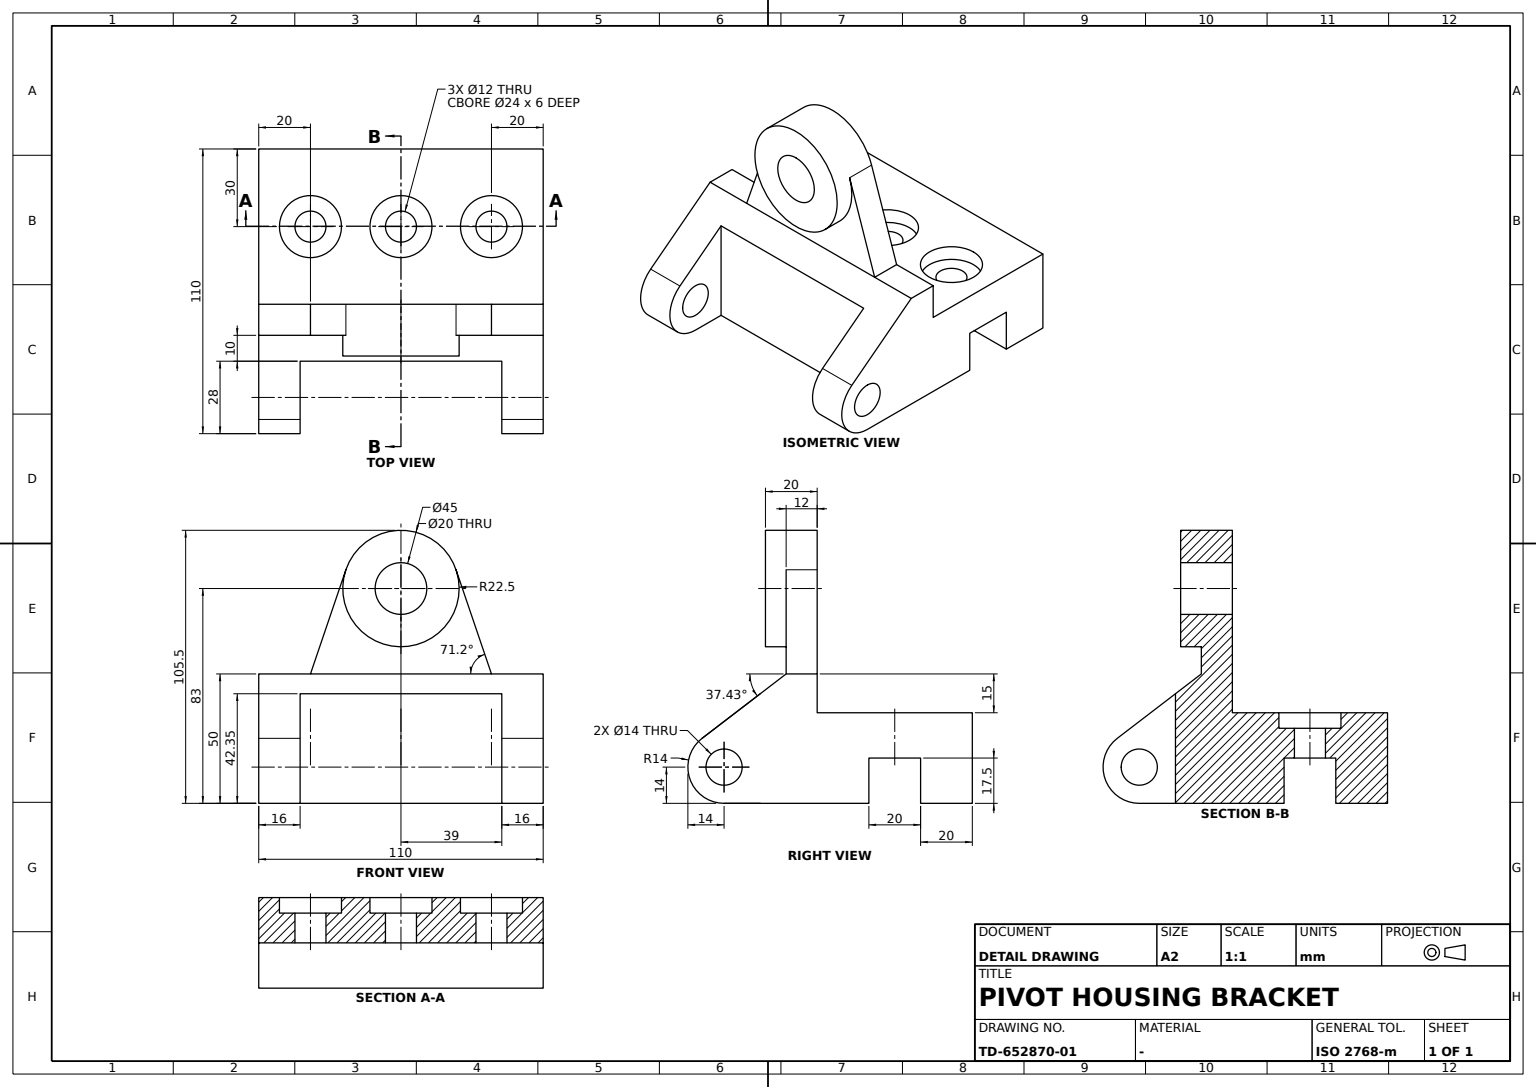
ISO-10303-21;
HEADER;
FILE_DESCRIPTION((''),'2;1');
FILE_NAME('','',(''),(''),'','','');
FILE_SCHEMA(('AUTOMOTIVE_DESIGN'));
ENDSEC;
DATA;
#1=APPLICATION_CONTEXT('');
#2=PRODUCT_CONTEXT('',#1,'mechanical');
#3=PRODUCT('','','',(#2));
#4=PRODUCT_DEFINITION_FORMATION('','',#3);
#5=PRODUCT_DEFINITION_CONTEXT('',#1,'design');
#6=PRODUCT_DEFINITION('','',#4,#5);
#7=PRODUCT_DEFINITION_SHAPE('','',#6);
#8=(LENGTH_UNIT()NAMED_UNIT(*)SI_UNIT(.MILLI.,.METRE.));
#9=(NAMED_UNIT(*)PLANE_ANGLE_UNIT()SI_UNIT($,.RADIAN.));
#10=(NAMED_UNIT(*)SI_UNIT($,.STERADIAN.)SOLID_ANGLE_UNIT());
#11=UNCERTAINTY_MEASURE_WITH_UNIT(LENGTH_MEASURE(0.005),#8,'distance_accuracy_value','');
#12=(GEOMETRIC_REPRESENTATION_CONTEXT(3)GLOBAL_UNCERTAINTY_ASSIGNED_CONTEXT((#11))GLOBAL_UNIT_ASSIGNED_CONTEXT((#8,#9,#10))REPRESENTATION_CONTEXT('',''));
#13=CARTESIAN_POINT('',(35.,-32.,32.5));
#14=VERTEX_POINT('',#13);
#15=CARTESIAN_POINT('',(-35.,-32.,32.5));
#16=VERTEX_POINT('',#15);
#17=DIRECTION('',(-1.,0.,0.));
#18=VECTOR('',#17,1000.);
#19=LINE('',#13,#18);
#20=EDGE_CURVE('',#14,#16,#19,.T.);
#21=ORIENTED_EDGE('',*,*,#20,.F.);
#22=CARTESIAN_POINT('',(21.299957,-32.,72.749954));
#23=VERTEX_POINT('',#22);
#24=DIRECTION('',(0.32222019,0.,-0.94666475));
#25=VECTOR('',#24,1000.);
#26=LINE('',#22,#25);
#27=EDGE_CURVE('',#23,#14,#26,.T.);
#28=ORIENTED_EDGE('',*,*,#27,.F.);
#29=CARTESIAN_POINT('',(-21.299957,-32.,72.749954));
#30=VERTEX_POINT('',#29);
#31=CARTESIAN_POINT('',(0.,-32.,65.5));
#32=DIRECTION('',(0.,1.,0.));
#33=DIRECTION('',(0.,0.,1.));
#34=AXIS2_PLACEMENT_3D('',#31,#32,#33);
#35=CIRCLE('',#34,22.5);
#36=EDGE_CURVE('',#30,#23,#35,.F.);
#37=ORIENTED_EDGE('',*,*,#36,.F.);
#38=DIRECTION('',(0.32222019,0.,0.94666475));
#39=VECTOR('',#38,1000.);
#40=LINE('',#15,#39);
#41=EDGE_CURVE('',#16,#30,#40,.T.);
#42=ORIENTED_EDGE('',*,*,#41,.F.);
#43=EDGE_LOOP('',(#21,#28,#37,#42));
#44=FACE_BOUND('',#43,.T.);
#45=PLANE('',#34);
#46=ADVANCED_FACE('',(#44),#45,.F.);
#47=CARTESIAN_POINT('',(55.,40.,17.5));
#48=VERTEX_POINT('',#47);
#49=CARTESIAN_POINT('',(-55.,40.,17.5));
#50=VERTEX_POINT('',#49);
#51=LINE('',#47,#18);
#52=EDGE_CURVE('',#48,#50,#51,.T.);
#53=ORIENTED_EDGE('',*,*,#52,.F.);
#54=CARTESIAN_POINT('',(55.,40.,-17.5));
#55=VERTEX_POINT('',#54);
#56=DIRECTION('',(0.,0.,-1.));
#57=VECTOR('',#56,1000.);
#58=LINE('',#47,#57);
#59=EDGE_CURVE('',#48,#55,#58,.T.);
#60=ORIENTED_EDGE('',*,*,#59,.T.);
#61=CARTESIAN_POINT('',(-55.,40.,-17.5));
#62=VERTEX_POINT('',#61);
#63=LINE('',#54,#18);
#64=EDGE_CURVE('',#55,#62,#63,.T.);
#65=ORIENTED_EDGE('',*,*,#64,.T.);
#66=LINE('',#49,#57);
#67=EDGE_CURVE('',#50,#62,#66,.T.);
#68=ORIENTED_EDGE('',*,*,#67,.F.);
#69=EDGE_LOOP('',(#53,#60,#65,#68));
#70=FACE_BOUND('',#69,.T.);
#71=AXIS2_PLACEMENT_3D('',#47,#32,#33);
#72=PLANE('',#71);
#73=ADVANCED_FACE('',(#70),#72,.T.);
#74=CARTESIAN_POINT('',(22.5,-40.,65.5));
#75=VERTEX_POINT('',#74);
#76=CARTESIAN_POINT('',(0.,-40.,65.5));
#77=DIRECTION('',(0.,-1.,0.));
#78=DIRECTION('',(1.,0.,0.));
#79=AXIS2_PLACEMENT_3D('',#76,#77,#78);
#80=CIRCLE('',#79,22.5);
#81=EDGE_CURVE('',#75,#75,#80,.T.);
#82=ORIENTED_EDGE('',*,*,#81,.T.);
#83=EDGE_LOOP('',(#82));
#84=FACE_BOUND('',#83,.T.);
#85=CARTESIAN_POINT('',(0.,-40.,75.5));
#86=VERTEX_POINT('',#85);
#87=AXIS2_PLACEMENT_3D('',#76,#32,#33);
#88=CIRCLE('',#87,10.);
#89=EDGE_CURVE('',#86,#86,#88,.T.);
#90=ORIENTED_EDGE('',*,*,#89,.T.);
#91=EDGE_LOOP('',(#90));
#92=FACE_BOUND('',#91,.T.);
#93=AXIS2_PLACEMENT_3D('',#76,#77,#56);
#94=PLANE('',#93);
#95=ADVANCED_FACE('',(#84,#92),#94,.T.);
#96=CARTESIAN_POINT('',(0.,-20.,75.5));
#97=VERTEX_POINT('',#96);
#98=CARTESIAN_POINT('',(0.,-20.,65.5));
#99=AXIS2_PLACEMENT_3D('',#98,#32,#33);
#100=CIRCLE('',#99,10.);
#101=EDGE_CURVE('',#97,#97,#100,.T.);
#102=ORIENTED_EDGE('',*,*,#101,.T.);
#103=EDGE_LOOP('',(#102));
#104=FACE_BOUND('',#103,.T.);
#105=ORIENTED_EDGE('',*,*,#89,.F.);
#106=EDGE_LOOP('',(#105));
#107=FACE_BOUND('',#106,.T.);
#108=CYLINDRICAL_SURFACE('',#87,10.);
#109=ADVANCED_FACE('',(#104,#107),#108,.F.);
#110=CARTESIAN_POINT('',(-21.299957,-20.,72.749954));
#111=VERTEX_POINT('',#110);
#112=VECTOR('',#32,1000.);
#113=LINE('',#29,#112);
#114=EDGE_CURVE('',#30,#111,#113,.T.);
#115=ORIENTED_EDGE('',*,*,#114,.F.);
#116=ORIENTED_EDGE('',*,*,#36,.T.);
#117=CARTESIAN_POINT('',(21.299957,-20.,72.749954));
#118=VERTEX_POINT('',#117);
#119=LINE('',#22,#112);
#120=EDGE_CURVE('',#23,#118,#119,.T.);
#121=ORIENTED_EDGE('',*,*,#120,.T.);
#122=AXIS2_PLACEMENT_3D('',#98,#32,#78);
#123=CIRCLE('',#122,22.5);
#124=EDGE_CURVE('',#111,#118,#123,.T.);
#125=ORIENTED_EDGE('',*,*,#124,.F.);
#126=EDGE_LOOP('',(#115,#116,#121,#125));
#127=FACE_BOUND('',#126,.T.);
#128=ORIENTED_EDGE('',*,*,#81,.F.);
#129=EDGE_LOOP('',(#128));
#130=FACE_BOUND('',#129,.T.);
#131=CYLINDRICAL_SURFACE('',#34,22.5);
#132=ADVANCED_FACE('',(#127,#130),#131,.T.);
#133=CARTESIAN_POINT('',(-39.,-42.,24.84594));
#134=VERTEX_POINT('',#133);
#135=CARTESIAN_POINT('',(-39.,-64.509212,7.617253));
#136=VERTEX_POINT('',#135);
#137=DIRECTION('',(0.,-0.794089474,-0.607800878));
#138=VECTOR('',#137,1000.);
#139=LINE('',#135,#138);
#140=EDGE_CURVE('',#134,#136,#139,.T.);
#141=ORIENTED_EDGE('',*,*,#140,.T.);
#142=CARTESIAN_POINT('',(-39.,-56.,-17.5));
#143=VERTEX_POINT('',#142);
#144=CARTESIAN_POINT('',(-39.,-56.,-3.5));
#145=AXIS2_PLACEMENT_3D('',#144,#17,#77);
#146=CIRCLE('',#145,14.);
#147=EDGE_CURVE('',#136,#143,#146,.F.);
#148=ORIENTED_EDGE('',*,*,#147,.T.);
#149=CARTESIAN_POINT('',(-39.,-42.,-17.5));
#150=VERTEX_POINT('',#149);
#151=CARTESIAN_POINT('',(-39.,-20.,-17.5));
#152=LINE('',#151,#112);
#153=EDGE_CURVE('',#143,#150,#152,.T.);
#154=ORIENTED_EDGE('',*,*,#153,.T.);
#155=CARTESIAN_POINT('',(-39.,-42.,55.));
#156=LINE('',#155,#57);
#157=EDGE_CURVE('',#150,#134,#156,.F.);
#158=ORIENTED_EDGE('',*,*,#157,.T.);
#159=EDGE_LOOP('',(#141,#148,#154,#158));
#160=FACE_BOUND('',#159,.T.);
#161=CARTESIAN_POINT('',(-39.,-63.,-3.5));
#162=VERTEX_POINT('',#161);
#163=CIRCLE('',#145,7.);
#164=EDGE_CURVE('',#162,#162,#163,.T.);
#165=ORIENTED_EDGE('',*,*,#164,.T.);
#166=EDGE_LOOP('',(#165));
#167=FACE_BOUND('',#166,.T.);
#168=CARTESIAN_POINT('',(-39.,-72.,55.));
#169=AXIS2_PLACEMENT_3D('',#168,#17,#77);
#170=PLANE('',#169);
#171=ADVANCED_FACE('',(#160,#167),#170,.F.);
#172=CARTESIAN_POINT('',(6.,10.,0.));
#173=VERTEX_POINT('',#172);
#174=CARTESIAN_POINT('',(0.,10.,0.));
#175=AXIS2_PLACEMENT_3D('',#174,#33,#78);
#176=CIRCLE('',#175,6.);
#177=EDGE_CURVE('',#173,#173,#176,.T.);
#178=ORIENTED_EDGE('',*,*,#177,.F.);
#179=EDGE_LOOP('',(#178));
#180=FACE_BOUND('',#179,.T.);
#181=CARTESIAN_POINT('',(0.,16.,11.5));
#182=VERTEX_POINT('',#181);
#183=CARTESIAN_POINT('',(0.,10.,11.5));
#184=AXIS2_PLACEMENT_3D('',#183,#56,#32);
#185=CIRCLE('',#184,6.);
#186=EDGE_CURVE('',#182,#182,#185,.F.);
#187=ORIENTED_EDGE('',*,*,#186,.T.);
#188=EDGE_LOOP('',(#187));
#189=FACE_BOUND('',#188,.T.);
#190=CARTESIAN_POINT('',(0.,10.,-65.061518));
#191=AXIS2_PLACEMENT_3D('',#190,#56,#32);
#192=CYLINDRICAL_SURFACE('',#191,6.);
#193=ADVANCED_FACE('',(#180,#189),#192,.F.);
#194=CARTESIAN_POINT('',(35.,-20.,32.5));
#195=VERTEX_POINT('',#194);
#196=LINE('',#13,#112);
#197=EDGE_CURVE('',#14,#195,#196,.T.);
#198=ORIENTED_EDGE('',*,*,#197,.T.);
#199=LINE('',#117,#25);
#200=EDGE_CURVE('',#118,#195,#199,.T.);
#201=ORIENTED_EDGE('',*,*,#200,.F.);
#202=ORIENTED_EDGE('',*,*,#120,.F.);
#203=ORIENTED_EDGE('',*,*,#27,.T.);
#204=EDGE_LOOP('',(#198,#201,#202,#203));
#205=FACE_BOUND('',#204,.T.);
#206=DIRECTION('',(0.94666475,0.,0.32222019));
#207=AXIS2_PLACEMENT_3D('',#22,#206,#24);
#208=PLANE('',#207);
#209=ADVANCED_FACE('',(#205),#208,.T.);
#210=CARTESIAN_POINT('',(55.,20.,0.));
#211=VERTEX_POINT('',#210);
#212=CARTESIAN_POINT('',(-55.,20.,0.));
#213=VERTEX_POINT('',#212);
#214=CARTESIAN_POINT('',(75.,20.,0.));
#215=LINE('',#214,#18);
#216=EDGE_CURVE('',#211,#213,#215,.T.);
#217=ORIENTED_EDGE('',*,*,#216,.T.);
#218=CARTESIAN_POINT('',(-55.,20.,-17.5));
#219=VERTEX_POINT('',#218);
#220=LINE('',#212,#57);
#221=EDGE_CURVE('',#219,#213,#220,.F.);
#222=ORIENTED_EDGE('',*,*,#221,.F.);
#223=CARTESIAN_POINT('',(55.,20.,-17.5));
#224=VERTEX_POINT('',#223);
#225=CARTESIAN_POINT('',(75.,20.,-17.5));
#226=LINE('',#225,#18);
#227=EDGE_CURVE('',#224,#219,#226,.T.);
#228=ORIENTED_EDGE('',*,*,#227,.F.);
#229=LINE('',#210,#57);
#230=EDGE_CURVE('',#224,#211,#229,.F.);
#231=ORIENTED_EDGE('',*,*,#230,.T.);
#232=EDGE_LOOP('',(#217,#222,#228,#231));
#233=FACE_BOUND('',#232,.T.);
#234=AXIS2_PLACEMENT_3D('',#225,#32,#33);
#235=PLANE('',#234);
#236=ADVANCED_FACE('',(#233),#235,.F.);
#237=CARTESIAN_POINT('',(-29.,10.,0.));
#238=VERTEX_POINT('',#237);
#239=CARTESIAN_POINT('',(-35.,10.,0.));
#240=AXIS2_PLACEMENT_3D('',#239,#33,#78);
#241=CIRCLE('',#240,6.);
#242=EDGE_CURVE('',#238,#238,#241,.T.);
#243=ORIENTED_EDGE('',*,*,#242,.F.);
#244=EDGE_LOOP('',(#243));
#245=FACE_BOUND('',#244,.T.);
#246=CARTESIAN_POINT('',(-41.,10.,11.5));
#247=VERTEX_POINT('',#246);
#248=CARTESIAN_POINT('',(-35.,10.,11.5));
#249=AXIS2_PLACEMENT_3D('',#248,#56,#17);
#250=CIRCLE('',#249,6.);
#251=EDGE_CURVE('',#247,#247,#250,.F.);
#252=ORIENTED_EDGE('',*,*,#251,.T.);
#253=EDGE_LOOP('',(#252));
#254=FACE_BOUND('',#253,.T.);
#255=CARTESIAN_POINT('',(-35.,10.,-58.75745));
#256=AXIS2_PLACEMENT_3D('',#255,#56,#17);
#257=CYLINDRICAL_SURFACE('',#256,6.);
#258=ADVANCED_FACE('',(#245,#254),#257,.F.);
#259=CARTESIAN_POINT('',(-35.,-20.,32.5));
#260=VERTEX_POINT('',#259);
#261=CARTESIAN_POINT('',(-55.,-20.,32.5));
#262=VERTEX_POINT('',#261);
#263=CARTESIAN_POINT('',(55.,-20.,32.5));
#264=LINE('',#263,#18);
#265=EDGE_CURVE('',#260,#262,#264,.T.);
#266=ORIENTED_EDGE('',*,*,#265,.T.);
#267=CARTESIAN_POINT('',(-55.,-32.,32.5));
#268=VERTEX_POINT('',#267);
#269=LINE('',#267,#112);
#270=EDGE_CURVE('',#268,#262,#269,.T.);
#271=ORIENTED_EDGE('',*,*,#270,.F.);
#272=CARTESIAN_POINT('',(55.,-32.,32.5));
#273=LINE('',#272,#18);
#274=EDGE_CURVE('',#16,#268,#273,.T.);
#275=ORIENTED_EDGE('',*,*,#274,.F.);
#276=LINE('',#15,#112);
#277=EDGE_CURVE('',#16,#260,#276,.T.);
#278=ORIENTED_EDGE('',*,*,#277,.T.);
#279=EDGE_LOOP('',(#266,#271,#275,#278));
#280=FACE_BOUND('',#279,.T.);
#281=AXIS2_PLACEMENT_3D('',#272,#33,#78);
#282=PLANE('',#281);
#283=ADVANCED_FACE('',(#280),#282,.T.);
#284=CARTESIAN_POINT('',(-55.,0.,0.));
#285=VERTEX_POINT('',#284);
#286=CARTESIAN_POINT('',(-55.,0.,-17.5));
#287=VERTEX_POINT('',#286);
#288=VECTOR('',#33,1000.);
#289=LINE('',#284,#288);
#290=EDGE_CURVE('',#285,#287,#289,.F.);
#291=ORIENTED_EDGE('',*,*,#290,.F.);
#292=CARTESIAN_POINT('',(55.,0.,0.));
#293=VERTEX_POINT('',#292);
#294=CARTESIAN_POINT('',(-75.,0.,0.));
#295=VECTOR('',#78,1000.);
#296=LINE('',#294,#295);
#297=EDGE_CURVE('',#285,#293,#296,.T.);
#298=ORIENTED_EDGE('',*,*,#297,.T.);
#299=CARTESIAN_POINT('',(55.,0.,-17.5));
#300=VERTEX_POINT('',#299);
#301=LINE('',#292,#288);
#302=EDGE_CURVE('',#293,#300,#301,.F.);
#303=ORIENTED_EDGE('',*,*,#302,.T.);
#304=CARTESIAN_POINT('',(-75.,0.,-17.5));
#305=LINE('',#304,#295);
#306=EDGE_CURVE('',#287,#300,#305,.T.);
#307=ORIENTED_EDGE('',*,*,#306,.F.);
#308=EDGE_LOOP('',(#291,#298,#303,#307));
#309=FACE_BOUND('',#308,.T.);
#310=AXIS2_PLACEMENT_3D('',#304,#77,#78);
#311=PLANE('',#310);
#312=ADVANCED_FACE('',(#309),#311,.F.);
#313=CARTESIAN_POINT('',(0.,22.,11.5));
#314=VERTEX_POINT('',#313);
#315=CIRCLE('',#184,12.);
#316=EDGE_CURVE('',#314,#314,#315,.F.);
#317=ORIENTED_EDGE('',*,*,#316,.F.);
#318=EDGE_LOOP('',(#317));
#319=FACE_BOUND('',#318,.T.);
#320=CARTESIAN_POINT('',(0.,22.,17.5));
#321=VERTEX_POINT('',#320);
#322=CARTESIAN_POINT('',(0.,10.,17.5));
#323=AXIS2_PLACEMENT_3D('',#322,#56,#32);
#324=CIRCLE('',#323,12.);
#325=EDGE_CURVE('',#321,#321,#324,.T.);
#326=ORIENTED_EDGE('',*,*,#325,.F.);
#327=EDGE_LOOP('',(#326));
#328=FACE_BOUND('',#327,.T.);
#329=CYLINDRICAL_SURFACE('',#323,12.);
#330=ADVANCED_FACE('',(#319,#328),#329,.F.);
#331=CARTESIAN_POINT('',(39.,-49.,-3.5));
#332=VERTEX_POINT('',#331);
#333=CARTESIAN_POINT('',(39.,-56.,-3.5));
#334=AXIS2_PLACEMENT_3D('',#333,#78,#32);
#335=CIRCLE('',#334,7.);
#336=EDGE_CURVE('',#332,#332,#335,.T.);
#337=ORIENTED_EDGE('',*,*,#336,.T.);
#338=EDGE_LOOP('',(#337));
#339=FACE_BOUND('',#338,.T.);
#340=CARTESIAN_POINT('',(39.,-42.,-17.5));
#341=VERTEX_POINT('',#340);
#342=CARTESIAN_POINT('',(39.,-42.,24.84594));
#343=VERTEX_POINT('',#342);
#344=CARTESIAN_POINT('',(39.,-42.,55.));
#345=LINE('',#344,#57);
#346=EDGE_CURVE('',#341,#343,#345,.F.);
#347=ORIENTED_EDGE('',*,*,#346,.F.);
#348=CARTESIAN_POINT('',(39.,-56.,-17.5));
#349=VERTEX_POINT('',#348);
#350=CARTESIAN_POINT('',(39.,-20.,-17.5));
#351=VECTOR('',#77,1000.);
#352=LINE('',#350,#351);
#353=EDGE_CURVE('',#341,#349,#352,.T.);
#354=ORIENTED_EDGE('',*,*,#353,.T.);
#355=CARTESIAN_POINT('',(39.,-64.509212,7.617253));
#356=VERTEX_POINT('',#355);
#357=CIRCLE('',#334,14.);
#358=EDGE_CURVE('',#349,#356,#357,.F.);
#359=ORIENTED_EDGE('',*,*,#358,.T.);
#360=DIRECTION('',(0.,0.794089474,0.607800878));
#361=VECTOR('',#360,1000.);
#362=LINE('',#355,#361);
#363=EDGE_CURVE('',#356,#343,#362,.T.);
#364=ORIENTED_EDGE('',*,*,#363,.T.);
#365=EDGE_LOOP('',(#347,#354,#359,#364));
#366=FACE_BOUND('',#365,.T.);
#367=AXIS2_PLACEMENT_3D('',#344,#78,#32);
#368=PLANE('',#367);
#369=ADVANCED_FACE('',(#339,#366),#368,.F.);
#370=CARTESIAN_POINT('',(41.,10.,0.));
#371=VERTEX_POINT('',#370);
#372=CARTESIAN_POINT('',(35.,10.,0.));
#373=AXIS2_PLACEMENT_3D('',#372,#33,#78);
#374=CIRCLE('',#373,6.);
#375=EDGE_CURVE('',#371,#371,#374,.T.);
#376=ORIENTED_EDGE('',*,*,#375,.F.);
#377=EDGE_LOOP('',(#376));
#378=FACE_BOUND('',#377,.T.);
#379=CARTESIAN_POINT('',(35.,16.,11.5));
#380=VERTEX_POINT('',#379);
#381=CARTESIAN_POINT('',(35.,10.,11.5));
#382=AXIS2_PLACEMENT_3D('',#381,#56,#32);
#383=CIRCLE('',#382,6.);
#384=EDGE_CURVE('',#380,#380,#383,.F.);
#385=ORIENTED_EDGE('',*,*,#384,.T.);
#386=EDGE_LOOP('',(#385));
#387=FACE_BOUND('',#386,.T.);
#388=CARTESIAN_POINT('',(35.,10.,-58.75745));
#389=AXIS2_PLACEMENT_3D('',#388,#56,#32);
#390=CYLINDRICAL_SURFACE('',#389,6.);
#391=ADVANCED_FACE('',(#378,#387),#390,.F.);
#392=CARTESIAN_POINT('',(-55.,-56.,3.5));
#393=VERTEX_POINT('',#392);
#394=CARTESIAN_POINT('',(-55.,-56.,-3.5));
#395=AXIS2_PLACEMENT_3D('',#394,#17,#33);
#396=CIRCLE('',#395,7.);
#397=EDGE_CURVE('',#393,#393,#396,.T.);
#398=ORIENTED_EDGE('',*,*,#397,.T.);
#399=EDGE_LOOP('',(#398));
#400=FACE_BOUND('',#399,.T.);
#401=ORIENTED_EDGE('',*,*,#164,.F.);
#402=EDGE_LOOP('',(#401));
#403=FACE_BOUND('',#402,.T.);
#404=CARTESIAN_POINT('',(55.,-56.,-3.5));
#405=AXIS2_PLACEMENT_3D('',#404,#17,#33);
#406=CYLINDRICAL_SURFACE('',#405,7.);
#407=ADVANCED_FACE('',(#400,#403),#406,.F.);
#408=ORIENTED_EDGE('',*,*,#316,.T.);
#409=EDGE_LOOP('',(#408));
#410=FACE_BOUND('',#409,.T.);
#411=ORIENTED_EDGE('',*,*,#186,.F.);
#412=EDGE_LOOP('',(#411));
#413=FACE_BOUND('',#412,.T.);
#414=PLANE('',#184);
#415=ADVANCED_FACE('',(#410,#413),#414,.F.);
#416=ORIENTED_EDGE('',*,*,#41,.T.);
#417=ORIENTED_EDGE('',*,*,#114,.T.);
#418=LINE('',#259,#39);
#419=EDGE_CURVE('',#260,#111,#418,.T.);
#420=ORIENTED_EDGE('',*,*,#419,.F.);
#421=ORIENTED_EDGE('',*,*,#277,.F.);
#422=EDGE_LOOP('',(#416,#417,#420,#421));
#423=FACE_BOUND('',#422,.T.);
#424=DIRECTION('',(-0.94666475,0.,0.32222019));
#425=AXIS2_PLACEMENT_3D('',#15,#424,#38);
#426=PLANE('',#425);
#427=ADVANCED_FACE('',(#423),#426,.T.);
#428=VERTEX_POINT('',#263);
#429=CARTESIAN_POINT('',(55.,-20.,17.5));
#430=VERTEX_POINT('',#429);
#431=LINE('',#263,#57);
#432=EDGE_CURVE('',#428,#430,#431,.T.);
#433=ORIENTED_EDGE('',*,*,#432,.T.);
#434=CARTESIAN_POINT('',(-55.,-20.,17.5));
#435=VERTEX_POINT('',#434);
#436=LINE('',#429,#295);
#437=EDGE_CURVE('',#435,#430,#436,.T.);
#438=ORIENTED_EDGE('',*,*,#437,.F.);
#439=LINE('',#261,#57);
#440=EDGE_CURVE('',#262,#435,#439,.T.);
#441=ORIENTED_EDGE('',*,*,#440,.F.);
#442=ORIENTED_EDGE('',*,*,#265,.F.);
#443=ORIENTED_EDGE('',*,*,#419,.T.);
#444=ORIENTED_EDGE('',*,*,#124,.T.);
#445=ORIENTED_EDGE('',*,*,#200,.T.);
#446=EDGE_CURVE('',#428,#195,#264,.T.);
#447=ORIENTED_EDGE('',*,*,#446,.F.);
#448=EDGE_LOOP('',(#433,#438,#441,#442,#443,#444,#445,#447));
#449=FACE_BOUND('',#448,.T.);
#450=ORIENTED_EDGE('',*,*,#101,.F.);
#451=EDGE_LOOP('',(#450));
#452=FACE_BOUND('',#451,.T.);
#453=AXIS2_PLACEMENT_3D('',#263,#32,#33);
#454=PLANE('',#453);
#455=ADVANCED_FACE('',(#449,#452),#454,.T.);
#456=LINE('',#284,#112);
#457=EDGE_CURVE('',#213,#285,#456,.F.);
#458=ORIENTED_EDGE('',*,*,#457,.F.);
#459=ORIENTED_EDGE('',*,*,#216,.F.);
#460=LINE('',#292,#112);
#461=EDGE_CURVE('',#211,#293,#460,.F.);
#462=ORIENTED_EDGE('',*,*,#461,.T.);
#463=ORIENTED_EDGE('',*,*,#297,.F.);
#464=EDGE_LOOP('',(#458,#459,#462,#463));
#465=FACE_BOUND('',#464,.T.);
#466=ORIENTED_EDGE('',*,*,#375,.T.);
#467=EDGE_LOOP('',(#466));
#468=FACE_BOUND('',#467,.T.);
#469=ORIENTED_EDGE('',*,*,#242,.T.);
#470=EDGE_LOOP('',(#469));
#471=FACE_BOUND('',#470,.T.);
#472=ORIENTED_EDGE('',*,*,#177,.T.);
#473=EDGE_LOOP('',(#472));
#474=FACE_BOUND('',#473,.T.);
#475=CARTESIAN_POINT('',(0.,0.,0.));
#476=AXIS2_PLACEMENT_3D('',#475,#33,#78);
#477=PLANE('',#476);
#478=ADVANCED_FACE('',(#465,#468,#471,#474),#477,.F.);
#479=CARTESIAN_POINT('',(-55.,-56.,-17.5));
#480=VERTEX_POINT('',#479);
#481=CARTESIAN_POINT('',(-55.,-20.,-17.5));
#482=LINE('',#481,#351);
#483=EDGE_CURVE('',#287,#480,#482,.T.);
#484=ORIENTED_EDGE('',*,*,#483,.F.);
#485=ORIENTED_EDGE('',*,*,#306,.T.);
#486=CARTESIAN_POINT('',(55.,-56.,-17.5));
#487=VERTEX_POINT('',#486);
#488=CARTESIAN_POINT('',(55.,-20.,-17.5));
#489=LINE('',#488,#351);
#490=EDGE_CURVE('',#300,#487,#489,.T.);
#491=ORIENTED_EDGE('',*,*,#490,.T.);
#492=LINE('',#486,#18);
#493=EDGE_CURVE('',#487,#349,#492,.T.);
#494=ORIENTED_EDGE('',*,*,#493,.T.);
#495=ORIENTED_EDGE('',*,*,#353,.F.);
#496=CARTESIAN_POINT('',(55.,-42.,-17.5));
#497=LINE('',#496,#295);
#498=EDGE_CURVE('',#150,#341,#497,.T.);
#499=ORIENTED_EDGE('',*,*,#498,.F.);
#500=ORIENTED_EDGE('',*,*,#153,.F.);
#501=EDGE_CURVE('',#143,#480,#492,.T.);
#502=ORIENTED_EDGE('',*,*,#501,.T.);
#503=EDGE_LOOP('',(#484,#485,#491,#494,#495,#499,#500,#502));
#504=FACE_BOUND('',#503,.T.);
#505=AXIS2_PLACEMENT_3D('',#488,#56,#17);
#506=PLANE('',#505);
#507=ADVANCED_FACE('',(#504),#506,.T.);
#508=CARTESIAN_POINT('',(55.,-64.509212,7.617253));
#509=VERTEX_POINT('',#508);
#510=AXIS2_PLACEMENT_3D('',#404,#17,#32);
#511=CIRCLE('',#510,14.);
#512=EDGE_CURVE('',#487,#509,#511,.T.);
#513=ORIENTED_EDGE('',*,*,#512,.F.);
#514=ORIENTED_EDGE('',*,*,#490,.F.);
#515=ORIENTED_EDGE('',*,*,#302,.F.);
#516=ORIENTED_EDGE('',*,*,#461,.F.);
#517=ORIENTED_EDGE('',*,*,#230,.F.);
#518=LINE('',#54,#351);
#519=EDGE_CURVE('',#55,#224,#518,.T.);
#520=ORIENTED_EDGE('',*,*,#519,.F.);
#521=ORIENTED_EDGE('',*,*,#59,.F.);
#522=CARTESIAN_POINT('',(55.,-56.,17.5));
#523=LINE('',#522,#112);
#524=EDGE_CURVE('',#430,#48,#523,.T.);
#525=ORIENTED_EDGE('',*,*,#524,.F.);
#526=ORIENTED_EDGE('',*,*,#432,.F.);
#527=VERTEX_POINT('',#272);
#528=LINE('',#272,#112);
#529=EDGE_CURVE('',#527,#428,#528,.T.);
#530=ORIENTED_EDGE('',*,*,#529,.F.);
#531=LINE('',#508,#361);
#532=EDGE_CURVE('',#509,#527,#531,.T.);
#533=ORIENTED_EDGE('',*,*,#532,.F.);
#534=EDGE_LOOP('',(#513,#514,#515,#516,#517,#520,#521,#525,#526,#530,#533));
#535=FACE_BOUND('',#534,.T.);
#536=CARTESIAN_POINT('',(55.,-56.,3.5));
#537=VERTEX_POINT('',#536);
#538=CIRCLE('',#405,7.);
#539=EDGE_CURVE('',#537,#537,#538,.T.);
#540=ORIENTED_EDGE('',*,*,#539,.T.);
#541=EDGE_LOOP('',(#540));
#542=FACE_BOUND('',#541,.T.);
#543=PLANE('',#405);
#544=ADVANCED_FACE('',(#535,#542),#543,.F.);
#545=CARTESIAN_POINT('',(-55.,-64.509212,7.617253));
#546=VERTEX_POINT('',#545);
#547=LINE('',#545,#361);
#548=EDGE_CURVE('',#546,#268,#547,.T.);
#549=ORIENTED_EDGE('',*,*,#548,.F.);
#550=LINE('',#508,#18);
#551=EDGE_CURVE('',#136,#546,#550,.T.);
#552=ORIENTED_EDGE('',*,*,#551,.F.);
#553=ORIENTED_EDGE('',*,*,#140,.F.);
#554=CARTESIAN_POINT('',(55.,-42.,24.84594));
#555=LINE('',#554,#18);
#556=EDGE_CURVE('',#343,#134,#555,.T.);
#557=ORIENTED_EDGE('',*,*,#556,.F.);
#558=ORIENTED_EDGE('',*,*,#363,.F.);
#559=EDGE_CURVE('',#509,#356,#550,.T.);
#560=ORIENTED_EDGE('',*,*,#559,.F.);
#561=ORIENTED_EDGE('',*,*,#532,.T.);
#562=EDGE_CURVE('',#527,#14,#273,.T.);
#563=ORIENTED_EDGE('',*,*,#562,.T.);
#564=ORIENTED_EDGE('',*,*,#20,.T.);
#565=ORIENTED_EDGE('',*,*,#274,.T.);
#566=EDGE_LOOP('',(#549,#552,#553,#557,#558,#560,#561,#563,#564,#565));
#567=FACE_BOUND('',#566,.T.);
#568=DIRECTION('',(0.,-0.607800878,0.794089474));
#569=AXIS2_PLACEMENT_3D('',#508,#568,#137);
#570=PLANE('',#569);
#571=ADVANCED_FACE('',(#567),#570,.T.);
#572=ORIENTED_EDGE('',*,*,#501,.F.);
#573=ORIENTED_EDGE('',*,*,#147,.F.);
#574=ORIENTED_EDGE('',*,*,#551,.T.);
#575=AXIS2_PLACEMENT_3D('',#394,#17,#32);
#576=CIRCLE('',#575,14.);
#577=EDGE_CURVE('',#480,#546,#576,.T.);
#578=ORIENTED_EDGE('',*,*,#577,.F.);
#579=EDGE_LOOP('',(#572,#573,#574,#578));
#580=FACE_BOUND('',#579,.T.);
#581=CYLINDRICAL_SURFACE('',#405,14.);
#582=ADVANCED_FACE('',(#580),#581,.T.);
#583=CARTESIAN_POINT('',(-47.,10.,17.5));
#584=VERTEX_POINT('',#583);
#585=CARTESIAN_POINT('',(-35.,10.,17.5));
#586=AXIS2_PLACEMENT_3D('',#585,#56,#17);
#587=CIRCLE('',#586,12.);
#588=EDGE_CURVE('',#584,#584,#587,.T.);
#589=ORIENTED_EDGE('',*,*,#588,.F.);
#590=EDGE_LOOP('',(#589));
#591=FACE_BOUND('',#590,.T.);
#592=CARTESIAN_POINT('',(-47.,10.,11.5));
#593=VERTEX_POINT('',#592);
#594=CIRCLE('',#249,12.);
#595=EDGE_CURVE('',#593,#593,#594,.F.);
#596=ORIENTED_EDGE('',*,*,#595,.F.);
#597=EDGE_LOOP('',(#596));
#598=FACE_BOUND('',#597,.T.);
#599=CYLINDRICAL_SURFACE('',#586,12.);
#600=ADVANCED_FACE('',(#591,#598),#599,.F.);
#601=CARTESIAN_POINT('',(35.,22.,11.5));
#602=VERTEX_POINT('',#601);
#603=CIRCLE('',#382,12.);
#604=EDGE_CURVE('',#602,#602,#603,.F.);
#605=ORIENTED_EDGE('',*,*,#604,.F.);
#606=EDGE_LOOP('',(#605));
#607=FACE_BOUND('',#606,.T.);
#608=CARTESIAN_POINT('',(35.,22.,17.5));
#609=VERTEX_POINT('',#608);
#610=CARTESIAN_POINT('',(35.,10.,17.5));
#611=AXIS2_PLACEMENT_3D('',#610,#56,#32);
#612=CIRCLE('',#611,12.);
#613=EDGE_CURVE('',#609,#609,#612,.T.);
#614=ORIENTED_EDGE('',*,*,#613,.F.);
#615=EDGE_LOOP('',(#614));
#616=FACE_BOUND('',#615,.T.);
#617=CYLINDRICAL_SURFACE('',#611,12.);
#618=ADVANCED_FACE('',(#607,#616),#617,.F.);
#619=ORIENTED_EDGE('',*,*,#67,.T.);
#620=LINE('',#61,#351);
#621=EDGE_CURVE('',#62,#219,#620,.T.);
#622=ORIENTED_EDGE('',*,*,#621,.T.);
#623=ORIENTED_EDGE('',*,*,#221,.T.);
#624=ORIENTED_EDGE('',*,*,#457,.T.);
#625=ORIENTED_EDGE('',*,*,#290,.T.);
#626=ORIENTED_EDGE('',*,*,#483,.T.);
#627=ORIENTED_EDGE('',*,*,#577,.T.);
#628=ORIENTED_EDGE('',*,*,#548,.T.);
#629=ORIENTED_EDGE('',*,*,#270,.T.);
#630=ORIENTED_EDGE('',*,*,#440,.T.);
#631=CARTESIAN_POINT('',(-55.,-56.,17.5));
#632=LINE('',#631,#112);
#633=EDGE_CURVE('',#435,#50,#632,.T.);
#634=ORIENTED_EDGE('',*,*,#633,.T.);
#635=EDGE_LOOP('',(#619,#622,#623,#624,#625,#626,#627,#628,#629,#630,#634));
#636=FACE_BOUND('',#635,.T.);
#637=ORIENTED_EDGE('',*,*,#397,.F.);
#638=EDGE_LOOP('',(#637));
#639=FACE_BOUND('',#638,.T.);
#640=PLANE('',#395);
#641=ADVANCED_FACE('',(#636,#639),#640,.T.);
#642=ORIENTED_EDGE('',*,*,#512,.T.);
#643=ORIENTED_EDGE('',*,*,#559,.T.);
#644=ORIENTED_EDGE('',*,*,#358,.F.);
#645=ORIENTED_EDGE('',*,*,#493,.F.);
#646=EDGE_LOOP('',(#642,#643,#644,#645));
#647=FACE_BOUND('',#646,.T.);
#648=ADVANCED_FACE('',(#647),#581,.T.);
#649=ORIENTED_EDGE('',*,*,#604,.T.);
#650=EDGE_LOOP('',(#649));
#651=FACE_BOUND('',#650,.T.);
#652=ORIENTED_EDGE('',*,*,#384,.F.);
#653=EDGE_LOOP('',(#652));
#654=FACE_BOUND('',#653,.T.);
#655=PLANE('',#382);
#656=ADVANCED_FACE('',(#651,#654),#655,.F.);
#657=ORIENTED_EDGE('',*,*,#346,.T.);
#658=ORIENTED_EDGE('',*,*,#556,.T.);
#659=ORIENTED_EDGE('',*,*,#157,.F.);
#660=ORIENTED_EDGE('',*,*,#498,.T.);
#661=EDGE_LOOP('',(#657,#658,#659,#660));
#662=FACE_BOUND('',#661,.T.);
#663=AXIS2_PLACEMENT_3D('',#155,#32,#33);
#664=PLANE('',#663);
#665=ADVANCED_FACE('',(#662),#664,.F.);
#666=ORIENTED_EDGE('',*,*,#595,.T.);
#667=EDGE_LOOP('',(#666));
#668=FACE_BOUND('',#667,.T.);
#669=ORIENTED_EDGE('',*,*,#251,.F.);
#670=EDGE_LOOP('',(#669));
#671=FACE_BOUND('',#670,.T.);
#672=PLANE('',#249);
#673=ADVANCED_FACE('',(#668,#671),#672,.F.);
#674=ORIENTED_EDGE('',*,*,#524,.T.);
#675=ORIENTED_EDGE('',*,*,#52,.T.);
#676=ORIENTED_EDGE('',*,*,#633,.F.);
#677=ORIENTED_EDGE('',*,*,#437,.T.);
#678=EDGE_LOOP('',(#674,#675,#676,#677));
#679=FACE_BOUND('',#678,.T.);
#680=ORIENTED_EDGE('',*,*,#588,.T.);
#681=EDGE_LOOP('',(#680));
#682=FACE_BOUND('',#681,.T.);
#683=ORIENTED_EDGE('',*,*,#613,.T.);
#684=EDGE_LOOP('',(#683));
#685=FACE_BOUND('',#684,.T.);
#686=ORIENTED_EDGE('',*,*,#325,.T.);
#687=EDGE_LOOP('',(#686));
#688=FACE_BOUND('',#687,.T.);
#689=AXIS2_PLACEMENT_3D('',#522,#33,#77);
#690=PLANE('',#689);
#691=ADVANCED_FACE('',(#679,#682,#685,#688),#690,.T.);
#692=ORIENTED_EDGE('',*,*,#64,.F.);
#693=ORIENTED_EDGE('',*,*,#519,.T.);
#694=ORIENTED_EDGE('',*,*,#227,.T.);
#695=ORIENTED_EDGE('',*,*,#621,.F.);
#696=EDGE_LOOP('',(#692,#693,#694,#695));
#697=FACE_BOUND('',#696,.T.);
#698=AXIS2_PLACEMENT_3D('',#54,#56,#32);
#699=PLANE('',#698);
#700=ADVANCED_FACE('',(#697),#699,.T.);
#701=ORIENTED_EDGE('',*,*,#446,.T.);
#702=ORIENTED_EDGE('',*,*,#197,.F.);
#703=ORIENTED_EDGE('',*,*,#562,.F.);
#704=ORIENTED_EDGE('',*,*,#529,.T.);
#705=EDGE_LOOP('',(#701,#702,#703,#704));
#706=FACE_BOUND('',#705,.T.);
#707=ADVANCED_FACE('',(#706),#282,.T.);
#708=ORIENTED_EDGE('',*,*,#336,.F.);
#709=EDGE_LOOP('',(#708));
#710=FACE_BOUND('',#709,.T.);
#711=ORIENTED_EDGE('',*,*,#539,.F.);
#712=EDGE_LOOP('',(#711));
#713=FACE_BOUND('',#712,.T.);
#714=ADVANCED_FACE('',(#710,#713),#406,.F.);
#715=CLOSED_SHELL('',(#46,#73,#95,#109,#132,#171,#193,#209,#236,#258,#283,#312,#330,#369,#391,#407,#415,#427,#455,#478,#507,#544,#571,#582,#600,#618,#641,#648,#656,#665,#673,#691,#700,#707,#714));
#716=MANIFOLD_SOLID_BREP('',#715);
#717=ADVANCED_BREP_SHAPE_REPRESENTATION('',(#716),#12);
#718=SHAPE_DEFINITION_REPRESENTATION(#7,#717);
ENDSEC;
END-ISO-10303-21;
